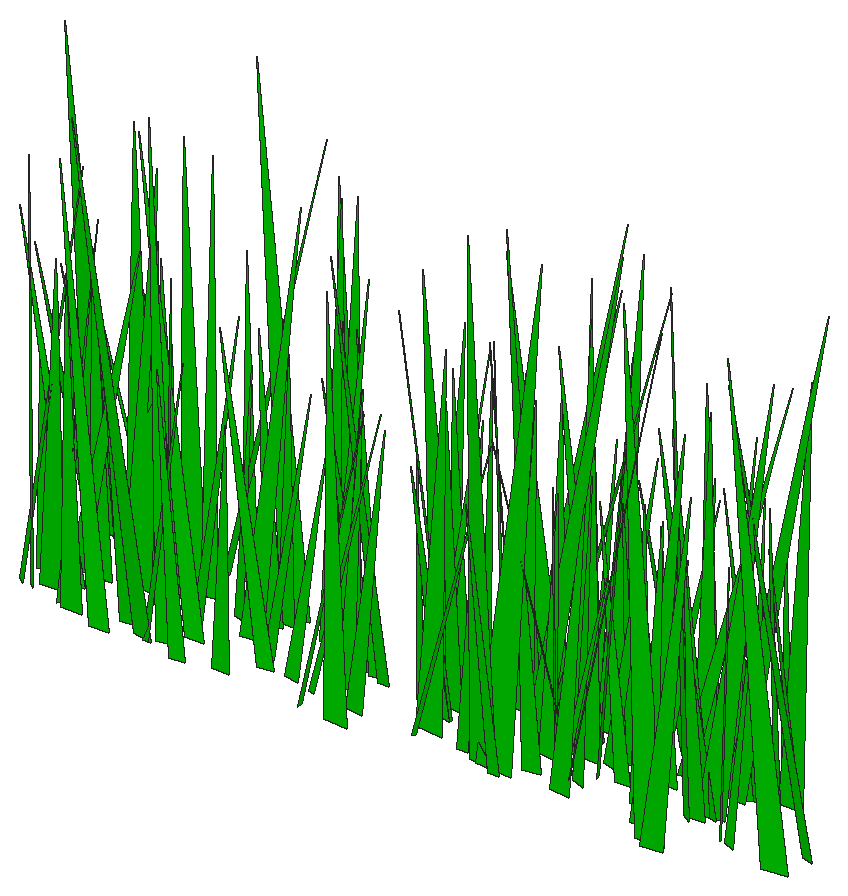
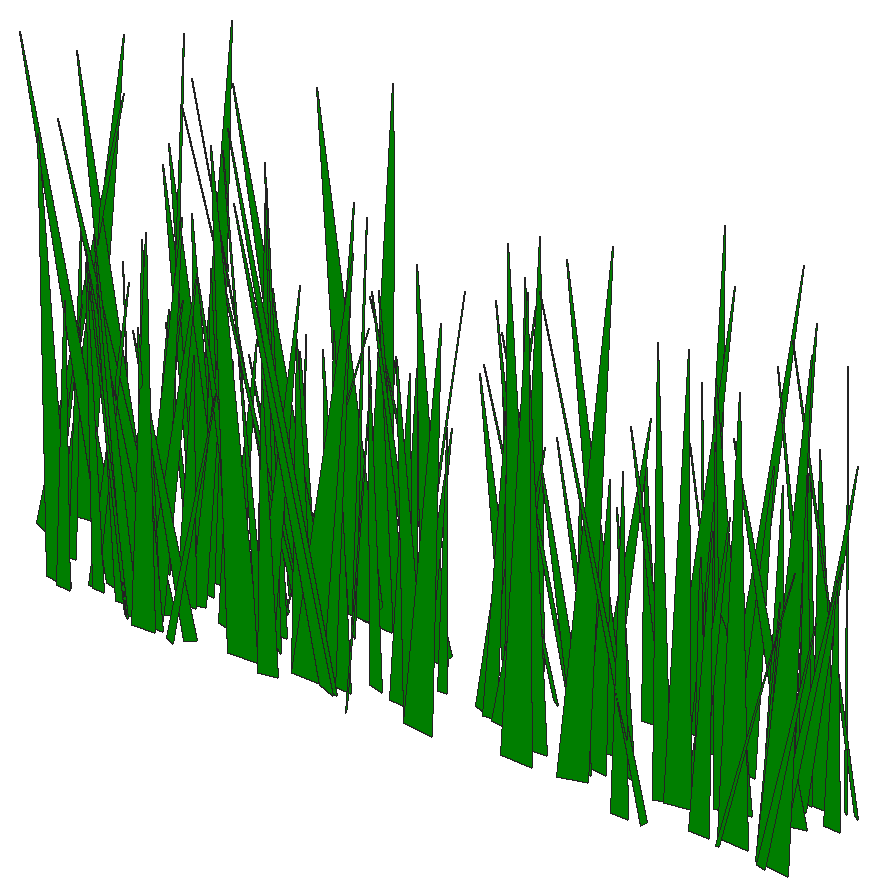
# SketchUp Ruby script. Lengths in inches.
U = 1.inch
M = Sketchup.active_model
def pt(a) = Geom::Point3d.new(a.map { |v| v * U })
def face(e, loops, mat)
  f = e.add_face(loops[0].map { |a| pt(a) })
  loops[1..].each { |l| e.add_face(l.map { |a| pt(a) }).erase! }
  f.material = f.back_material = mat if mat
  f
end
# faces: each face lists its corners as indices into pts; further lists are holes
def faces(e, pts, list, mat = nil) = list.each { |f| face(e, (f[0].is_a?(Array) ? f : [f]).map { |l| l.map { |i| pts[i] } }, mat) }
# xy, xz, yz: faces in a plane at the given z, y or x. An outline is a flat list of corners, or four numbers for a rectangle; further outlines are holes
def ring(l) = l.size == 4 ? [[l[0], l[1]], [l[2], l[1]], [l[2], l[3]], [l[0], l[3]]] : l.each_slice(2).to_a
def flat(e, list, mat, &to3) = list.each { |f| face(e, (f[0].is_a?(Array) ? f : [f]).map { |l| ring(l).map { |u, v| to3.(u, v) } }, mat) }
def xy(e, z, list, mat = nil) = flat(e, list, mat) { |x, y| [x, y, z] }
def xz(e, y, list, mat = nil) = flat(e, list, mat) { |x, z| [x, y, z] }
def yz(e, x, list, mat = nil) = flat(e, list, mat) { |y, z| [x, y, z] }
def lines(e, pts, list) = list.each { |a, b| e.add_line(pt(pts[a]), pt(pts[b])) }
# prism: a flat outline (further loops are holes) pulled along v
def prism(e, loops, v, mat = nil)
  f = face(e, loops, mat); d = Geom::Vector3d.new(v.map { |x| x * U })
  f.pushpull(f.normal.samedirection?(d) ? d.length : -d.length)
end
def box(e, o, s, mat = nil) = prism(e, [[o, [o[0] + s[0], o[1], o[2]], [o[0] + s[0], o[1] + s[1], o[2]], [o[0], o[1] + s[1], o[2]]]], [0, 0, s[2]], mat)
def at(x, y, z, deg = 0) = Geom::Transformation.translation(pt([x, y, z])) * Geom::Transformation.rotation(ORIGIN, Z_AXIS, deg.degrees)
def axes(o, x, y, z) = Geom::Transformation.new([*x, 0, *y, 0, *z, 0, *pt(o).to_a, 1])
def part(name) = M.definitions.add(name)
# library, detail: a bought-in or finely detailed component or shape, given as its bounding box
def library(name, o, s) = part(name).tap { |d| box(d.entities, o, s) }
def detail(e, o, s) = box(e.add_group.entities, o, s)
def put(e, d, t, mat = nil) = e.add_instance(d, t).tap { |i| i.material = mat if mat }
def group(e, t, mat = nil) = e.add_group.tap { |g| g.transformation = t; g.material = mat if mat }.entities
root = M.entities
M.materials.add("[Color G06]").color = [0, 204, 0]
c1 = part("fur_instance\#9")
p = [[0.8125,0,1.79],[0.67,-0.02,1.48],[0,-0.11,0],[0,0.11,0]]
faces(c1.entities,p,[[0,1,2,3]])
put(root,c1,axes([12.68,25.51,4.28],[-2.58079,-0.22105,0.23118],[-1.58479,0.36049,0.07739],[0.15892,0.00513,4.52603]),"[Color G06]")
put(root,c1,axes([12.4,25.38,4.28],[-2.23715,-0.72313,1.7638],[-5.3063,0.3155,-0.17472],[0.35771,0.15767,8.43914]),"[Color G06]")
put(root,c1,axes([13.08,24.23,4.28],[-2.99043,-0.24438,0.38519],[-1.76383,0.41731,-0.1732],[0.16347,0.03214,5.17749]),"[Color G06]")
put(root,c1,axes([12.49,22.61,4.28],[-0.76002,0.31444,1.91894],[2.5806,0.11111,0.19159],[0.27146,-0.1759,3.55126]),"[Color G06]")
put(root,c1,axes([12.77,21.65,4.28],[-4.34302,-0.10976,2.90334],[-0.81638,0.6626,0.14972],[1.93048,0.03328,6.595]),"[Color G06]")
put(root,c1,axes([13.875,22.36,4.28],[-3.64114,0.27988,0.76512],[2.03033,0.51083,0.11743],[0.41004,-0.04412,6.21283]),"[Color G06]")
put(root,c1,axes([13.24,24.91,4.28],[-2.58704,-0.10673,1.16227],[-0.76155,0.37645,0.18457],[0.78139,0.01355,4.02795]),"[Color G06]")
put(root,c1,axes([14.375,25.33,4.28],[-3.5454,0.01532,0.14252],[0.1143,0.49399,0.25293],[0.08996,-0.02401,5.29537]),"[Color G06]")
put(root,c1,axes([12.36,21.69,4.28],[4.81475,0.14386,1.48216],[1.06581,-0.68441,-0.10255],[-0.95492,-0.03851,7.35863]),"[Color G06]")
put(root,c1,axes([13.3,21.91,4.28],[0.8662,-0.54396,0.55951],[-3.91604,-0.12216,-0.10044],[-0.14703,0.04891,5.9713]),"[Color G06]")
put(root,c1,axes([14.1,23.17,4.28],[-0.2461,0.47302,2.02934],[3.65294,0.02766,0.24878],[-0.08063,-0.19043,5.07708]),"[Color G06]")
put(root,c1,axes([14,21.9,4.28],[-2.6208,-0.31097,2.43484],[-2.51081,0.39873,-0.18685],[1.15027,0.16181,5.13972]),"[Color G06]")
put(root,c1,axes([14.09,24.98,4.28],[0.86655,-0.64133,2.18452],[-4.80487,-0.13395,-0.25981],[-0.44942,0.19545,6.98992]),"[Color G06]")
put(root,c1,axes([14.57,21.21,4.28],[-1.16168,0.47141,1.14298],[3.45054,0.16792,-0.12222],[0.32755,-0.09704,5.34119]),"[Color G06]")
put(root,c1,axes([13.24,23.16,4.28],[3.37356,-0.33642,0.40529],[-2.42248,-0.47073,0.15604],[-0.15964,0.03386,6.19668]),"[Color G06]")
put(root,c1,axes([14,21.41,4.28],[4.33494,-0.07713,1.73883],[-0.52826,-0.62587,-0.24728],[-1.17491,-0.00316,6.52673]),"[Color G06]")
put(root,c1,axes([15.16,25.15,4.28],[-1.50893,0.39318,1.57553],[2.98537,0.21654,0.17894],[0.38591,-0.13781,4.77624]),"[Color G06]")
put(root,c1,axes([15.86,20.85,4.28],[-4.16823,0.4029,1.50917],[2.89858,0.59603,-0.39632],[0.98278,-0.04912,7.56966]),"[Color G06]")
put(root,c1,axes([15.17,23.47,4.28],[0.00072,0.67304,1.03435],[4.86961,0.00481,-0.36677],[0.24781,-0.09639,7.2043]),"[Color G06]")
put(root,c1,axes([15.41,23.67,4.28],[-1.61448,0.42687,2.79865],[3.45595,0.26206,-0.13834],[0.96631,-0.22404,5.17065]),"[Color G06]")
put(root,c1,axes([16.49,23.72,4.28],[-2.37795,0.33203,0.66043],[2.4057,0.33379,0.07154],[0.27806,-0.04835,5.02892]),"[Color G06]")
put(root,c1,axes([16.35,21.64,4.28],[-1.08312,-0.45865,0.82371],[-3.33493,0.14914,-0.25593],[0.00748,0.08047,5.16912]),"[Color G06]")
put(root,c1,axes([17.15,21.24,4.28],[-4.58798,-0.47318,1.34785],[-3.42985,0.64826,0.06428],[0.75094,0.0699,8.52853]),"[Color G06]")
put(root,c1,axes([16.05,24,4.28],[-1.4409,-0.27676,1.77687],[-2.22773,0.21867,-0.12272],[0.62424,0.14156,3.66352]),"[Color G06]")
put(root,c1,axes([16.64,24.25,4.28],[-2.90558,0.53592,2.25654],[3.99781,0.42953,-0.21997],[1.03314,-0.15489,7.19742]),"[Color G06]")
put(root,c1,axes([17.16,24.3,4.28],[3.97263,-0.2937,3.08032],[-2.37297,-0.60486,0.21096],[-1.74728,0.15369,6.71696]),"[Color G06]")
put(root,c1,axes([18.39,22.07,4.28],[-4.76529,0.38074,1.38592],[2.73437,0.67595,-0.33098],[0.91559,-0.03706,8.20167]),"[Color G06]")
put(root,c1,axes([17.54,25.6875,4.28],[2.53194,-0.3211,2.18017],[-2.45069,-0.3897,-0.23597],[-1.1935,0.11901,5.10966]),"[Color G06]")
put(root,c1,axes([17.87,21.41,4.28],[-4.7327,0.37873,2.97804],[2.87129,0.70412,-0.09391],[1.76139,-0.1302,8.15481]),"[Color G06]")
put(root,c1,axes([17.7,21.68,4.28],[-3.58689,-0.09548,2.5934],[-0.73884,0.55425,0.06156],[1.71288,0.03912,5.45733]),"[Color G06]")
put(root,c1,axes([17.32,21.17,4.28],[3.07615,0.14887,0.99614],[1.05552,-0.43884,0.2529],[-0.68544,-0.00768,4.85996]),"[Color G06]")
put(root,c1,axes([18.75,20.82,4.28],[-2.05132,0.32739,1.07442],[2.41009,0.29345,0.00642],[0.46967,-0.07589,4.65967]),"[Color G06]")
put(root,c1,axes([17.83,22.93,4.28],[3.1283,0.24498,1.17527],[1.8269,-0.44379,-0.23556],[-0.60597,-0.07326,5.35713]),"[Color G06]")
put(root,c1,axes([16.74,25.62,4.28],[5.60193,-0.04232,0.74118],[-0.31486,-0.78396,0.17318],[-0.48879,0.01994,8.38299]),"[Color G06]")
put(root,c1,axes([18.59,23.875,4.28],[2.3214,0.19888,1.43829],[1.52721,-0.34198,-0.07374],[-0.79242,-0.07645,4.07135]),"[Color G06]")
put(root,c1,axes([19.83,24.92,4.28],[-4.27045,0.60719,1.69426],[4.39062,0.60999,-0.39228],[0.98361,-0.08669,9.10683]),"[Color G06]")
put(root,c1,axes([19.66,24.11,4.28],[-0.98008,0.41811,1.32799],[3.1257,0.13512,0.26578],[0.10001,-0.12559,4.70717]),"[Color G06]")
put(root,c1,axes([19.89,24.41,4.28],[-1.05227,-0.34798,2.03672],[-2.7967,0.1632,-0.02445],[0.5126,0.17609,4.04757]),"[Color G06]")
put(root,c1,axes([21.06,22,4.28],[-2.82447,0.34707,0.52287],[2.50171,0.39528,0.04623],[0.24193,-0.0355,5.6263]),"[Color G06]")
put(root,c1,axes([20.12,21.1,4.28],[0.33565,-0.39016,0.88695],[-2.86012,-0.04533,0.12717],[0.01569,0.08357,4.20976]),"[Color G06]")
put(root,c1,axes([19.65,23.1,4.28],[3.98384,-0.45857,1.44894],[-3.35666,-0.56389,0.11456],[-0.69792,0.09444,7.71981]),"[Color G06]")
put(root,c1,axes([20.71,22.59,4.28],[2.57662,0.25955,0.73031],[1.88911,-0.36285,-0.07404],[-0.36671,-0.04556,4.75005]),"[Color G06]")
put(root,c1,axes([21.7,25.05,4.28],[-1.4153,0.61417,3.21267],[4.88185,0.20415,0.32065],[0.43169,-0.29516,6.90669]),"[Color G06]")
put(root,c1,axes([21.73,24.32,4.28],[2.40655,-0.57017,2.66097],[-4.3668,-0.35854,-0.00348],[-0.90523,0.21379,7.09096]),"[Color G06]")
put(root,c1,axes([22,22.01,4.28],[1.48445,0.32346,0.37017],[2.33212,-0.20677,-0.13511],[-0.05698,-0.0359,4.11377]),"[Color G06]")
put(root,c1,axes([23.37,23.74,4.28],[-2.22066,-0.34092,0.43581],[-2.45395,0.31092,0.00913],[0.20059,0.02952,4.93625]),"[Color G06]")
put(root,c1,axes([22.8,23.74,4.28],[-0.65561,-0.51872,1.48589],[-3.84469,0.09585,0.05469],[0.20982,0.13561,5.64501]),"[Color G06]")
put(root,c1,axes([22.71,23.62,4.28],[1.23632,0.69235,2.13739],[5.15103,-0.18122,0.0878],[-0.40472,-0.19144,7.64672]),"[Color G06]")
put(root,c1,axes([22.27,23.55,4.28],[3.97876,-0.2837,1.49486],[-2.04604,-0.57069,-0.27763],[-0.97642,0.03981,6.67311]),"[Color G06]")
put(root,c1,axes([24.25,23.41,4.28],[-4.00981,-0.30512,1.52001],[-2.28653,0.56834,-0.36824],[0.77055,0.09873,6.81721]),"[Color G06]")
put(root,c1,axes([23.81,23.61,4.28],[2.84786,-0.23391,2.84411],[-1.88947,-0.46179,-0.13664],[-1.69259,0.12195,4.9379]),"[Color G06]")
put(root,c1,axes([23.59,22.54,4.28],[2.36253,-0.31961,1.60844],[-2.43095,-0.34372,0.13005],[-0.70841,0.11362,4.91784]),"[Color G06]")
put(root,c1,axes([22.91,21.8,4.28],[3.44287,0.1597,0.26738],[1.14213,-0.48072,0.13361],[-0.19795,0.00397,5.42121]),"[Color G06]")
put(root,c1,axes([23.13,20.99,4.28],[3.73817,-0.02498,0.52876],[-0.15944,-0.52287,-0.31995],[-0.36309,-0.02759,5.58422]),"[Color G06]")
put(root,c1,axes([24.61,20.76,4.28],[-3.02629,0.48052,2.11359],[3.54934,0.44908,-0.37652],[1.12985,-0.12369,6.84401]),"[Color G06]")
put(root,c1,axes([24.94,25.35,4.28],[-0.19662,-0.62053,1.30164],[-4.52873,0.02079,-0.3897],[-0.22705,0.12275,6.64592]),"[Color G06]")
put(root,c1,axes([24.58,21.66,4.28],[1.73022,0.38873,0.91418],[2.84518,-0.24278,-0.1694],[-0.2244,-0.08091,4.90076]),"[Color G06]")
put(root,c1,axes([25.26,25.04,4.28],[1.17135,0.55486,0.54011],[3.98341,-0.16625,0.32295],[-0.30998,-0.03974,6.19093]),"[Color G06]")
put(root,c1,axes([25.74,23.28,4.28],[-2.12553,-0.23146,1.47091],[-1.70246,0.32105,0.30802],[0.90844,0.06011,4.01883]),"[Color G06]")
put(root,c1,axes([26.1875,24.55,4.28],[1.04246,-0.44971,1.82974],[-3.3968,-0.1649,-0.33292],[-0.60109,0.15193,5.05464]),"[Color G06]")
put(root,c1,axes([27.09,22.97,4.28],[-4.36809,-0.00774,1.35626],[-0.08417,0.62178,-0.19793],[0.90525,0.02047,6.52596]),"[Color G06]")
put(root,c1,axes([26.76,22.96,4.28],[-1.52717,-0.35078,0.22061],[-2.51254,0.21381,0.20233],[0.19238,0.00777,4.39363]),"[Color G06]")
put(root,c1,axes([26.75,23.52,4.28],[1.6176,0.35694,2.4164],[2.89647,-0.25686,0.02744],[-0.88128,-0.18903,4.52551]),"[Color G06]")
put(root,c1,axes([27.1875,25.74,4.28],[-3.56936,-0.02894,1.67368],[-0.29016,0.51986,-0.34978],[1.10132,0.04318,5.33222]),"[Color G06]")
put(root,c1,axes([25.9,23.84,4.28],[4.00316,-0.18911,1.00678],[-1.34843,-0.566,-0.23634],[-0.68894,0.00897,6.31259]),"[Color G06]")
put(root,c1,axes([27,22.08,4.28],[0.44169,0.59933,1.26079],[4.37991,-0.05984,-0.15997],[0.02227,-0.11854,6.45547]),"[Color G06]")
put(root,c1,axes([27.3,24.29,4.28],[-2.61971,-0.2727,2.54265],[-2.24567,0.40723,-0.15107],[1.29448,0.15458,4.88364]),"[Color G06]")
put(root,c1,axes([28.46,25.02,4.28],[-3.93698,-0.45766,2.26082],[-3.35904,0.57848,0.38612],[1.33291,0.10604,7.65079]),"[Color G06]")
put(root,c1,axes([29.14,25.05,4.28],[-2.55406,0.62871,0.617],[4.52716,0.35548,0.24998],[0.05738,-0.06159,7.74058]),"[Color G06]")
put(root,c1,axes([26.78,21.66,4.28],[3.83354,-0.02388,0.2631],[-0.17761,-0.53475,0.20541],[-0.16961,0.02026,5.73154]),"[Color G06]")
put(root,c1,axes([28.08,24.91,4.28],[1.96519,-0.44753,1.33823],[-3.26091,-0.2881,-0.3713],[-0.68434,0.08765,5.61219]),"[Color G06]")
put(root,c1,axes([28.36,24.71,4.28],[1.99378,-0.36999,1.86834],[-2.86514,-0.29078,0.21483],[-0.62746,0.1521,4.95571]),"[Color G06]")
put(root,c1,axes([28.45,21.8,4.28],[2.88011,0.31422,1.5198],[2.27522,-0.42206,0.39316],[-0.96706,-0.05716,5.45132]),"[Color G06]")
put(root,c1,axes([29.4375,21.51,4.28],[3.02404,0.58308,4.32334],[4.81958,-0.47823,-0.12104],[-1.61973,-0.3344,7.71154]),"[Color G06]")
put(root,c1,axes([29.67,22.31,4.28],[-4.17233,-0.12399,2.52898],[-1.04687,0.62222,-0.35372],[1.59933,0.08383,6.36605]),"[Color G06]")
put(root,c1,axes([29.37,24.91,4.28],[-0.8434,0.48153,1.42872],[3.55625,0.12922,-0.31349],[0.43742,-0.12208,5.30348]),"[Color G06]")
put(root,c1,axes([30.02,21.26,4.28],[-2.18859,-0.26053,1.07508],[-1.95084,0.31092,-0.21552],[0.44989,0.08081,4.29541]),"[Color G06]")
put(root,c1,axes([28.31,25.22,4.28],[4.60592,0.3594,0.4891],[2.56612,-0.64385,0.36913],[-0.4061,0.00785,7.87972]),"[Color G06]")
put(root,c1,axes([28.24,25.1875,4.28],[5.13842,0.44448,0.7598],[3.19391,-0.71942,0.09678],[-0.46623,-0.02967,9.03682]),"[Color G06]")
put(root,c1,axes([30.98,24.69,4.28],[2.65591,-0.28484,4.11456],[-2.75371,-0.46651,0.26055],[-2.04172,0.25866,5.0009]),"[Color G06]")
put(root,c1,axes([30.11,25.5625,4.28],[-0.05873,-0.44775,0.70357],[-3.23599,0.01304,0.3498],[0.2451,0.06485,4.78702]),"[Color G06]")
put(root,c1,axes([31.88,22.56,4.28],[-3.72195,-0.05584,0.09299],[-0.40293,0.51847,-0.26138],[0.04308,0.02518,5.58871]),"[Color G06]")
put(root,c1,axes([30.76,22.07,4.28],[-0.37155,0.40559,1.13639],[3.00144,0.04394,0.39038],[-0.1717,-0.10952,4.36504]),"[Color G06]")
put(root,c1,axes([29.86,21.47,4.28],[1.51695,0.84564,0.07172],[6.06453,-0.21153,-0.01816],[0.00014,-0.0069,9.34284]),"[Color G06]")
put(root,c1,axes([30.34,25.43,4.28],[2.91112,-0.17476,1.41506],[-1.33847,-0.42151,0.17066],[-0.82195,0.06744,4.73388]),"[Color G06]")
put(root,c1,axes([30.6,23.05,4.28],[-0.0462,0.37564,2.01845],[3.00409,0.02051,-0.28497],[0.23635,-0.18731,4.01657]),"[Color G06]")
put(root,c1,axes([30.77,24.26,4.28],[-4.51228,-0.15619,3.60613],[-1.38321,0.70367,-0.36491],[2.27224,0.11818,6.93903]),"[Color G06]")
put(root,c1,axes([31.21,22.61,4.28],[-2.89144,0.00695,1.84323],[-0.04694,0.4371,-0.35391],[1.23339,0.03294,4.30759]),"[Color G06]")
put(root,c1,axes([29.95,23.27,4.28],[4.32457,0.59782,0.82462],[4.3101,-0.60462,-0.13796],[-0.32653,-0.06334,9.10005]),"[Color G06]")
put(root,c1,axes([31.49,23.64,4.28],[0.50417,0.64371,2.47861],[4.90277,-0.07325,-0.04239],[-0.15011,-0.23034,6.94015]),"[Color G06]")
put(root,c1,axes([31.23,25.21,4.28],[1.35239,0.72829,1.97574],[5.38685,-0.18566,-0.37491],[-0.081,-0.18729,8.05452]),"[Color G06]")
put(root,c1,axes([29.65,24.23,4.28],[5.9189,-0.02985,0.19546],[-0.21291,-0.82553,-0.08278],[-0.13269,-0.00706,8.85163]),"[Color G06]")
put(root,c1,axes([32.22,22.375,4.28],[2.79569,0.23759,1.88232],[1.88509,-0.41166,-0.28507],[-0.96727,-0.11558,4.88488]),"[Color G06]")
put(root,c1,axes([32.15,21.62,4.28],[1.0471,0.44488,0.82979],[3.2377,-0.14535,-0.17429],[-0.06073,-0.07865,5.0154]),"[Color G06]")
put(root,c1,axes([32.78,24.14,4.28],[-1.93452,-0.25775,1.66866],[-2.04202,0.28633,-0.20745],[0.70225,0.12257,3.99349]),"[Color G06]")
put(root,c1,axes([33.43,25.73,4.28],[-2.69005,-0.16617,0.63361],[-1.22062,0.37747,-0.20363],[0.33144,0.04147,4.39259]),"[Color G06]")
put(root,c1,axes([33.23,23.15,4.28],[-2.12309,0.30883,0.83956],[2.24273,0.30211,-0.09777],[0.43665,-0.05012,4.58428]),"[Color G06]")
put(root,c1,axes([31.97,21.89,4.28],[2.33039,0.20618,0.09321],[1.46867,-0.32421,0.36058],[-0.18175,0.02377,4.10903]),"[Color G06]")
put(root,c1,axes([32.43,23.02,4.28],[4.68368,0.02842,2.0922],[0.21848,-0.68157,-0.02905],[-1.39765,-0.01131,7.00667]),"[Color G06]")
put(root,c1,axes([32.31,23.73,4.28],[2.90019,0.31944,0.91884],[2.33872,-0.4077,-0.20668],[-0.3952,-0.06844,5.51978]),"[Color G06]")
put(root,c1,axes([34.05,23.71,4.28],[-3.24286,0.27607,1.3895],[2.02396,0.46666,-0.09959],[0.82913,-0.05938,5.67765]),"[Color G06]")
put(root,c1,axes([31.82,22.5,4.28],[5.59621,0.05194,0.96792],[0.39421,-0.78502,-0.25174],[-0.63464,-0.02959,8.37867]),"[Color G06]")
put(root,c1,axes([34.59,25.01,4.28],[-2.28332,-0.45316,0.51584],[-3.25027,0.32101,0.2577],[0.33985,0.02547,5.93036]),"[Color G06]")
put(root,c1,axes([32.99,25.38,4.28],[2.82377,-0.23101,0.3646],[-1.67195,-0.39266,0.34467],[-0.09287,0.04498,4.88087]),"[Color G06]")
put(root,c1,axes([34.32,23.05,4.28],[0.54048,0.31462,2.26549],[2.66329,-0.10438,0.24588],[-0.54334,-0.19866,3.4588]),"[Color G06]")
put(root,c1,axes([34.33,23.88,4.28],[-0.81279,0.40302,0.24292],[2.89329,0.11384,-0.07225],[0.0906,-0.01999,4.4865]),"[Color G06]")
put(root,c1,axes([34.42,25.68,4.28],[-1.74987,-0.50904,2.11013],[-3.83274,0.26657,0.28767],[0.79342,0.16505,6.04352]),"[Color G06]")
put(root,c1,axes([34.21,25.48,4.28],[0.66148,0.43191,1.21233],[3.20143,-0.09103,-0.17639],[-0.05015,-0.11409,4.73035]),"[Color G06]")
put(root,c1,axes([34.47,22.4375,4.28],[-0.44047,0.43252,1.95667],[3.35544,0.07142,-0.12641],[0.27476,-0.17888,4.68052]),"[Color G06]")
put(root,c1,axes([34.54,25.31,4.28],[1.58123,-0.51039,1.55028],[-3.76991,-0.23124,-0.15615],[-0.51033,0.12677,5.95697]),"[Color G06]")
put(root,c1,axes([34.68,23.09,4.28],[2.40638,0.18942,0.97258],[1.4025,-0.34415,-0.05153],[-0.54923,-0.0489,4.12964]),"[Color G06]")
put(root,c1,axes([35.96,23.3,4.28],[-2.25673,0.48997,1.02577],[3.56282,0.31847,0.03415],[0.35141,-0.08227,6.24124]),"[Color G06]")
put(root,c1,axes([36,20.95,4.28],[-3.89835,0.59879,2.09523],[4.37372,0.5649,-0.36807],[1.12905,-0.12086,8.66019]),"[Color G06]")
put(root,c1,axes([35.91,22.76,4.28],[5.07173,0.17185,4.05928],[1.43909,-0.79542,-0.14801],[-2.61238,-0.10454,7.79924]),"[Color G06]")
put(root,c1,axes([35.1,25.35,4.28],[3.62127,-0.20448,1.41494],[-1.51002,-0.51952,0.00787],[-0.87547,0.05025,5.83915]),"[Color G06]")
put(root,c1,axes([36.48,23.16,4.28],[-2.54133,-0.26204,0.6555],[-1.88187,0.35892,0.18543],[0.42685,0.02229,4.72017]),"[Color G06]")
put(root,c1,axes([35.28,21.55,4.28],[1.45197,0.64336,0.1875],[4.61532,-0.2025,-0.0179],[-0.02623,-0.01719,7.22889]),"[Color G06]")
put(root,c1,axes([35.24,25.4,4.28],[3.68778,0.10863,1.35651],[0.77478,-0.52948,0.16595],[-0.91125,-0.01057,5.63085]),"[Color G06]")
put(root,c1,axes([35.86,20.97,4.28],[0.81164,0.49417,1.03175],[3.60802,-0.11465,-0.03189],[-0.13294,-0.09451,5.4336]),"[Color G06]")
put(root,c1,axes([36.18,22.85,4.28],[-0.14958,-0.40842,0.453],[-2.94424,0.02012,-0.08744],[-0.04328,0.04262,4.38231]),"[Color G06]")
put(root,c1,axes([35.67,24.89,4.28],[1.26099,0.44798,0.8541],[3.26146,-0.17565,-0.17236],[-0.09988,-0.08009,5.15515]),"[Color G06]")
put(root,c1,axes([34.37,24.63,4.28],[4.95207,-0.26674,0.07394],[-1.91341,-0.69005,0.28197],[0.02187,0.02703,7.92921]),"[Color G06]")
put(root,c1,axes([36.99,24.67,4.28],[-2.96698,-0.23121,1.11756],[-1.67797,0.42493,0.14813],[0.70196,0.03849,5.07767]),"[Color G06]")
put(root,c1,axes([36.27,20.69,4.28],[1.87516,0.55134,0.05417],[3.94591,-0.26129,0.39266],[-0.25289,0.01114,6.5284]),"[Color G06]")
put(root,c1,axes([36.75,24.74,4.28],[-2.75801,0.15847,2.69483],[1.45741,0.44025,0.3578],[1.55515,-0.13154,4.44388]),"[Color G06]")
put(root,c1,axes([37.6,25.24,4.28],[-1.96856,-0.28487,1.90006],[-2.24431,0.29997,-0.02764],[0.86753,0.12961,4.24001]),"[Color G06]")
put(root,c1,axes([37.48,22.34,4.28],[2.86755,0.01719,1.69115],[0.07221,-0.42957,0.22812],[-1.13593,0.01609,4.28365]),"[Color G06]")
put(root,c1,axes([36.45,23.1875,4.28],[3.80688,-0.58489,0.28258],[-4.19247,-0.53146,-0.20225],[-0.2273,0.00683,8.46339]),"[Color G06]")
put(root,c1,axes([36.36,24.4,4.28],[4.7223,0.54576,0.50797],[3.90697,-0.66019,0.34911],[-0.41078,-0.0051,9.16007]),"[Color G06]")
put(root,c1,axes([38.64,24.53,4.28],[-2.72459,-0.1534,0.97876],[-1.1082,0.39011,0.13246],[0.64097,0.02243,4.38947]),"[Color G06]")
put(root,c1,axes([37.89,25.0625,4.28],[2.36489,0.56765,1.86395],[4.19204,-0.34521,0.19624],[-0.74369,-0.1408,7.03345]),"[Color G06]")
put(root,c1,axes([38.42,23.8125,4.28],[2.94114,0.1662,2.55892],[1.48132,-0.45696,-0.39369],[-1.46891,-0.12804,4.72661]),"[Color G06]")
put(root,c1,axes([37.89,22.24,4.28],[2.24382,0.21231,1.13997],[1.6216,-0.3201,-0.28126],[-0.51987,-0.08213,4.04292]),"[Color G06]")
put(root,c1,axes([40.18,22.97,4.28],[-4.72904,-0.29092,1.0828],[-2.12993,0.66391,-0.28786],[0.58389,0.06556,7.71978]),"[Color G06]")
put(root,c1,axes([39.86,21.85,4.28],[-3.72805,0.57792,1.43093],[4.2096,0.52674,0.06041],[0.60979,-0.10308,8.33118]),"[Color G06]")
